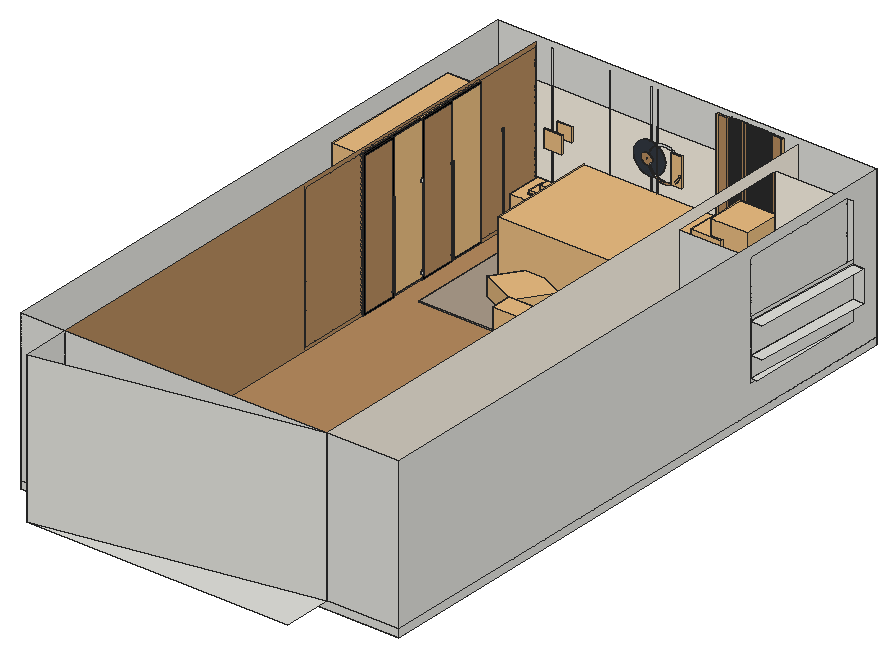
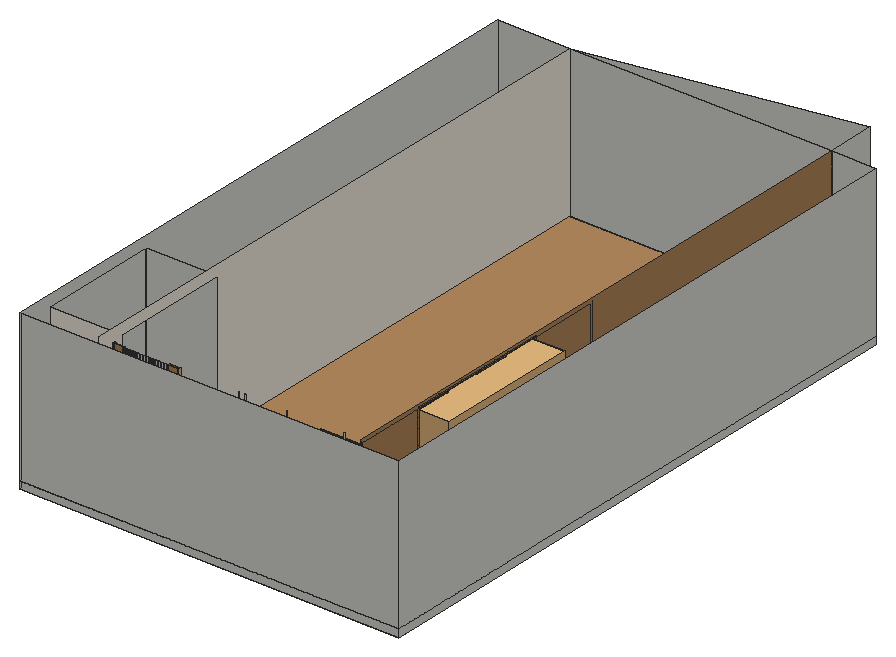
# SketchUp Ruby script. Lengths in inches.
U = 1.inch
M = Sketchup.active_model
def pt(a) = Geom::Point3d.new(a.map { |v| v * U })
def face(e, loops, mat)
  f = e.add_face(loops[0].map { |a| pt(a) })
  loops[1..].each { |l| e.add_face(l.map { |a| pt(a) }).erase! }
  f.material = f.back_material = mat if mat
  f
end
# faces: each face lists its corners as indices into pts; further lists are holes
def faces(e, pts, list, mat = nil) = list.each { |f| face(e, (f[0].is_a?(Array) ? f : [f]).map { |l| l.map { |i| pts[i] } }, mat) }
# xy, xz, yz: faces in a plane at the given z, y or x. An outline is a flat list of corners, or four numbers for a rectangle; further outlines are holes
def ring(l) = l.size == 4 ? [[l[0], l[1]], [l[2], l[1]], [l[2], l[3]], [l[0], l[3]]] : l.each_slice(2).to_a
def flat(e, list, mat, &to3) = list.each { |f| face(e, (f[0].is_a?(Array) ? f : [f]).map { |l| ring(l).map { |u, v| to3.(u, v) } }, mat) }
def xy(e, z, list, mat = nil) = flat(e, list, mat) { |x, y| [x, y, z] }
def xz(e, y, list, mat = nil) = flat(e, list, mat) { |x, z| [x, y, z] }
def yz(e, x, list, mat = nil) = flat(e, list, mat) { |y, z| [x, y, z] }
def lines(e, pts, list) = list.each { |a, b| e.add_line(pt(pts[a]), pt(pts[b])) }
# prism: a flat outline (further loops are holes) pulled along v
def prism(e, loops, v, mat = nil)
  f = face(e, loops, mat); d = Geom::Vector3d.new(v.map { |x| x * U })
  f.pushpull(f.normal.samedirection?(d) ? d.length : -d.length)
end
def box(e, o, s, mat = nil) = prism(e, [[o, [o[0] + s[0], o[1], o[2]], [o[0] + s[0], o[1] + s[1], o[2]], [o[0], o[1] + s[1], o[2]]]], [0, 0, s[2]], mat)
def at(x, y, z, deg = 0) = Geom::Transformation.translation(pt([x, y, z])) * Geom::Transformation.rotation(ORIGIN, Z_AXIS, deg.degrees)
def axes(o, x, y, z) = Geom::Transformation.new([*x, 0, *y, 0, *z, 0, *pt(o).to_a, 1])
def part(name) = M.definitions.add(name)
# library, detail: a bought-in or finely detailed component or shape, given as its bounding box
def library(name, o, s) = part(name).tap { |d| box(d.entities, o, s) }
def detail(e, o, s) = box(e.add_group.entities, o, s)
def put(e, d, t, mat = nil) = e.add_instance(d, t).tap { |i| i.material = mat if mat }
def group(e, t, mat = nil) = e.add_group.tap { |g| g.transformation = t; g.material = mat if mat }.entities
root = M.entities
M.materials.add("ChenZc-200606-DCZ97").color = [45, 44, 41]
M.materials.add("[0030_OldLace]").color = [253, 245, 230]
M.materials.add("[0110_LightSlateGray]").color = [51, 58, 66]
M.materials.add("[Color A01]").color = [254, 254, 199]
M.materials.add("[Color M09]").color = [0, 0, 0]
M.materials.add("[Metal_Aluminum_Anodized]1").color = [200, 209, 218]
M.materials.add("images-82sdfgh").color = [172, 157, 140]
M.materials.add("noyer1").color = [183, 140, 95]
c1 = library("组\#1",[0,0,0],[23.67,16.93,17.45])
c2 = library("Group22\#1",[-44.99,-22.85,-0.04],[43.91,45.38,19.57])
c3 = part("Untitled (22)")
g1 = group(c3.entities,at(0,0,0))
box(g1,[0,0,0],[170.08,120.47,0.79],"images-82sdfgh")
c4 = library("Group\#32",[-0.5,-0.5,0],[1,1.75,120])
c5 = library("Group\#33",[-0.5,-0.5,0],[1,1.9375,120])
c6 = library("Group\#27",[-9049.24,-32375.18,0],[19139.08,65939.34,16883.65])
c7 = part("27d7-b66a-ddc1-c0b1")
put(c7.entities,c6,at(0,0,0))
c8 = library("@05-床_01.第一季_组\#8",[0,0,0],[98.46,95.44,37.59])
c9 = library("Group80",[524.42,-273.19,102.05],[657.62,664.02,265.78])
c10 = library("Group73",[-242.83,-1394.05,-548.89],[487.85,171.35,750.9])
c11 = part("Дверь 1")
xy(c11.entities,0,[[0,-8.42,1.18,19.14]],"[Color M09]")
xy(c11.entities,0.79,[[0,-7.63,0.79,18.35],[0.79,-7.63,1.18,18.35]],"[Color M09]")
xy(c11.entities,95.67,[[0,-7.63,0.79,18.35]],"[Color M09]")
xy(c11.entities,95.67,[[0.79,-7.63,1.18,18.35]],"[Metal_Aluminum_Anodized]1")
xy(c11.entities,96.46,[[0,-8.42,1.18,19.14]],"[Color M09]")
xz(c11.entities,-8.42,[[0,0,1.18,96.46]],"[Color M09]")
xz(c11.entities,-7.63,[[0,0.79,0.79,95.67],[0.79,0.79,1.18,95.67]],"[Color M09]")
xz(c11.entities,18.35,[[0,0.79,0.79,95.67],[0.79,0.79,1.18,95.67]],"[Color M09]")
xz(c11.entities,19.14,[[0,0,1.18,96.46]],"[Metal_Aluminum_Anodized]1")
yz(c11.entities,0.79,[[-7.63,0.79,18.35,95.67]])
yz(c11.entities,1.18,[[[-8.42,0,19.14,96.46],[-7.63,0.79,18.35,95.67]]],"[Color M09]")
c12 = part("Group\#25")
put(c12.entities,c11,axes([0,38.03,0],[1,0,0],[0,1.05714,0],[0,0,1.11429]))
put(c12.entities,c11,axes([1.18,8.9,0],[1,0,0],[0,1.05714,0],[0,0,1.11429]))
c13 = library("dressing+1",[0,-1.62,0],[110.16,25.74,102.29])
c14 = part("POI-E1497-320-1917\#1")
xy(c14.entities,0,[[0,0,0.29,0.83],[7.21,0,7.5,0.83]])
xy(c14.entities,0.64,[[0.29,0.21,7.21,0.62]])
xy(c14.entities,0.875,[[0,0.21,7.5,0.62]])
xz(c14.entities,0.21,[[0,0.64,7.5,0.875]])
xz(c14.entities,0.62,[[0,0.64,7.5,0.875]])
yz(c14.entities,0,[[0,0,0.21,0.64,0.21,0.875,0.62,0.875,0.62,0.64,0.83,0]])
yz(c14.entities,0.29,[[0,0,0.83,0,0.62,0.64,0.21,0.64]])
yz(c14.entities,7.21,[[0,0,0.21,0.64,0.62,0.64,0.83,0]])
yz(c14.entities,7.5,[[0,0,0.83,0,0.62,0.64,0.62,0.875,0.21,0.875,0.21,0.64]])
p = [[0,0.21,0.64],[0,0,0],[0.29,0,0],[0.29,0.21,0.64],[7.21,0.21,0.64],[7.21,0,0],
  [7.5,0,0],[7.5,0.21,0.64],[0,0.83,0],[0,0.62,0.64],[0.29,0.62,0.64],[0.29,0.83,0],
  [7.5,0.83,0],[7.5,0.62,0.64],[7.21,0.62,0.64],[7.21,0.83,0]]
faces(c14.entities,p,[[0,1,2,3],[4,5,6,7],[8,9,10,11],[12,13,14,15]])
c15 = library("lamp",[0,0,0],[9.82,9.84,19.44])
c16 = library("17、植物花艺_花艺摆件_组\#4",[-0.13,-2.14,0],[21.63,21.46,31.4])
c17 = library("Pillow pair",[0,0,0],[18.27,24.9,18.7])
c18 = library("Group68\#1",[-167.83,-430.625,-1475.1875],[237.96,44,300])
c19 = library("Group69\#1",[-161.55,-462.88,-1311.24],[231.68,35.74,267.26])
c20 = library("Group67\#2",[-2553.52,-1371.9,-99.68],[199.61,250.46,199.36])
c21 = library("Omni Light",[-12,-12,-12],[24,24,24])
c22 = library("建立群組\#3",[-0.5,-0.5,0],[1.79,16.75,15.75])
c23 = library("Group\#29",[-0.5,-0.5,0],[8.5625,1,23.16])
c24 = library("建立群組\#4",[-0.5,-0.5,0],[1.79,16.75,15.75])
xy(root,-6,[[0,38.875,302.125,515.625]])
xy(root,0,[[35.9,0,244.6,38.875,244.6,0],[35.9,0,35.9,38.875,244.6,38.875],[0,38.875,35.9,38.875,35.9,508.85,48.54,508.85,48.54,508.97,48.84,508.97,48.84,508.85,94.41,508.85,94.41,508.97,94.71,508.97,94.71,508.85,127.66,508.85,127.66,508.97,127.96,508.97,127.96,508.85,132.6,508.85,132.6,508.97,132.9,508.97,132.9,508.85,180.6,508.85,180.6,509.54,189.03,509.54,189.03,509.85,190.82,509.85,190.82,510.22,191.46,510.22,191.46,509.85,193.25,509.85,193.25,510.22,193.9,510.22,193.9,509.85,195.69,509.85,195.69,510.22,196.34,510.22,196.34,509.85,198.13,509.85,198.13,510.22,198.78,510.22,198.78,509.85,200.57,509.85,200.57,510.22,201.21,510.22,201.21,509.85,203,509.85,203,510.22,203.53,510.22,203.53,509.85,205.32,509.85,205.32,510.22,205.84,510.22,205.84,509.85,207.63,509.85,207.63,510.22,208.15,510.22,208.15,509.85,209.94,509.85,209.94,510.22,210.46,510.22,210.46,509.85,212.25,509.85,212.25,510.22,212.78,510.22,212.78,509.85,214.57,509.85,214.57,510.22,215.09,510.22,215.09,509.85,216.88,509.85,216.88,510.22,217.4,510.22,217.4,509.85,219.19,509.85,219.19,510.22,219.71,510.22,219.71,509.85,221.5,509.85,221.5,510.22,222.03,510.22,222.03,509.85,223.82,509.85,223.82,510.22,224.53,510.22,224.53,509.54,232.6,509.54,232.6,508.85,244.6,508.85,244.6,38.875,302.125,38.875,302.125,515.625,0,515.625]])
xy(root,0,[[35.9,38.875,244.6,38.875,244.6,508.85,232.6,508.85,232.6,508.22,224.53,508.22,224.53,510.22,223.82,510.22,223.82,509.85,222.03,509.85,222.03,510.22,221.5,510.22,221.5,509.85,219.71,509.85,219.71,510.22,219.19,510.22,219.19,509.85,217.4,509.85,217.4,510.22,216.88,510.22,216.88,509.85,215.09,509.85,215.09,510.22,214.57,510.22,214.57,509.85,212.78,509.85,212.78,510.22,212.25,510.22,212.25,509.85,210.46,509.85,210.46,510.22,209.94,510.22,209.94,509.85,208.15,509.85,208.15,510.22,207.63,510.22,207.63,509.85,205.84,509.85,205.84,510.22,205.32,510.22,205.32,509.85,203.53,509.85,203.53,510.22,203,510.22,203,509.85,201.21,509.85,201.21,510.22,200.57,510.22,200.57,509.85,198.78,509.85,198.78,510.22,198.13,510.22,198.13,509.85,196.34,509.85,196.34,510.22,195.69,510.22,195.69,509.85,193.9,509.85,193.9,510.22,193.25,510.22,193.25,509.85,191.46,509.85,191.46,510.22,190.82,510.22,190.82,509.85,189.03,509.85,189.03,508.22,180.6,508.22,180.6,508.85,132.9,508.85,132.9,508.97,132.6,508.97,132.6,508.85,127.96,508.85,127.96,508.97,127.66,508.97,127.66,508.85,94.71,508.85,94.71,508.97,94.41,508.97,94.41,508.85,48.84,508.85,48.84,508.97,48.54,508.97,48.54,508.85,35.9,508.85],[180.6,508.22,189.03,509.54],[224.53,508.22,232.6,509.54]],"noyer1")
xy(root,3.11,[[2.53,335.23,35.9,450.62]],"noyer1")
xy(root,13.82,[[2.53,335.23,33.46,450.62]],"noyer1")
xy(root,14.91,[[2.53,335.23,33.46,450.62]],"noyer1")
xy(root,20.8125,[[244.6,390.22,244.91,486.22],[244.91,390.22,247.04,486.22]])
xy(root,21.9375,[[244.6,390.22,244.91,486.22],[244.91,390.22,247.04,486.22],[247.04,390.22,302.125,486.22]])
xy(root,25.1875,[[247.04,390.22,302.125,486.22],[302.125,390.22,302.125,486.22,306.875,486.22],[302.125,390.22,306.875,486.22,306.875,390.22]])
xy(root,37.91,[[2.53,335.23,33.46,450.62]],"noyer1")
xy(root,38.8,[[2.53,335.23,33.46,450.62]],"noyer1")
xy(root,41.64,[[311.68,389.75,302.125,390.22,306.875,486.22,316.43,485.75]])
xy(root,66.2,[[311.68,389.75,316.43,485.75,306.875,486.22,302.125,390.22]])
xz(root,38.875,[[0,-6,302.125,0],[0,0,35.9,120],[35.9,0,244.6,120],[244.6,0,302.125,120]])
xz(root,335.23,[[2.53,3.11,35.9,13.82],[2.53,13.82,33.46,14.91],[33.46,13.82,35.9,14.91],[2.53,14.91,35.9,37.91],[2.53,37.91,33.46,38.8],
  [33.46,37.91,35.9,38.8],[[2.53,38.8,35.9,85.91],[18.45,80.49,18.79,80.54,19.1,80.67,19.375,80.875,19.58,81.15,19.72,81.46,19.76,81.8,19.72,82.14,19.58,82.46,19.375,82.73,19.1,82.94,18.79,83.07,18.45,83.12,18.11,83.07,17.79,82.94,17.52,82.73,17.3125,82.46,17.18,82.14,17.14,81.8,17.18,81.46,17.3125,81.15,17.52,80.875,17.79,80.67,18.11,80.54]]])
xz(root,390.22,[[244.6,20.8125,244.91,21.9375],[244.91,20.8125,247.04,21.9375],[244.6,21.9375,244.6,25.1875,247.04,25.1875,246.71,25.04,246.41,24.86,246.12,24.66,245.84,24.43,245.59,24.17,245.37,23.9,245.17,23.61,245,23.3,244.85,22.97,244.74,22.63,244.65,22.29],[247.04,21.9375,302.125,25.1875],[244.6,25.1875,302.125,111.375]])
xz(root,450.62,[[2.53,3.11,35.9,13.82],[2.53,13.82,33.46,14.91],[33.46,13.82,35.9,14.91],[2.53,14.91,35.9,37.91],[2.53,37.91,33.46,38.8],
  [33.46,37.91,35.9,38.8],[[2.53,38.8,35.9,85.91],[18.45,80.49,18.11,80.54,17.79,80.67,17.52,80.875,17.3125,81.15,17.18,81.46,17.14,81.8,17.18,82.14,17.3125,82.46,17.52,82.73,17.79,82.94,18.11,83.07,18.45,83.12,18.79,83.07,19.1,82.94,19.375,82.73,19.58,82.46,19.72,82.14,19.76,81.8,19.72,81.46,19.58,81.15,19.375,80.875,19.1,80.67,18.79,80.54]]])
xz(root,486.22,[[244.6,20.8125,244.91,21.9375],[244.91,20.8125,247.04,21.9375],[247.04,21.9375,302.125,25.1875],[302.125,25.1875,306.875,111.375]])
xz(root,486.22,[[244.6,21.9375,244.65,22.29,244.74,22.63,244.85,22.97,245,23.3,245.17,23.61,245.37,23.9,245.59,24.17,245.84,24.43,246.12,24.66,246.41,24.86,246.71,25.04,247.04,25.1875,302.125,25.1875,302.125,111.375,244.6,111.375]],"[0030_OldLace]")
xz(root,506.41,[[[126.11,65.22,127.17,65.36,128.17,65.77,129.02,66.42,129.68,67.28,130.09,68.27,130.23,69.34,130.09,70.4,129.68,71.4,129.02,72.25,128.17,72.91,127.17,73.32,126.11,73.46,125.04,73.32,124.05,72.91,123.19,72.25,122.54,71.4,122.13,70.4,121.99,69.34,122.13,68.27,122.54,67.28,123.19,66.42,124.05,65.77,125.04,65.36],[125.18,68.71,126.7,70.22]]],"noyer1")
xz(root,507.33,[[126.11,65.22,125.04,65.36,124.05,65.77,123.19,66.42,122.54,67.28,122.13,68.27,121.99,69.34,122.13,70.4,122.54,71.4,123.19,72.25,124.05,72.91,125.04,73.32,126.11,73.46,126.26,73.4375,126.04,72.63,125.78,70.99,125.7,69.34,125.78,67.68,126.04,66.05,126.26,65.24],[126.26,65.24,126.04,66.05,125.78,67.68,125.7,69.34,125.78,70.99,126.04,72.63,126.26,73.4375,127.17,73.32,127.71,73.1,127.5,72.32,127.26,70.84,127.18,69.34,127.26,67.84,127.5,66.36,127.71,65.58,127.17,65.36],[127.71,65.58,127.5,66.36,127.26,67.84,127.18,69.34,127.26,70.84,127.5,72.32,127.71,73.1,128.17,72.91,129.02,72.25,129.68,71.4,130.09,70.4,130.23,69.34,130.09,68.27,129.68,67.28,129.02,66.42,128.17,65.77]])
xz(root,507.33,[[139.45,55.38,140.9,55.46,142.32,55.68,143.72,56.06,145.07,56.58,146.36,57.23,145.71,58.36,144.55,57.76,143.32,57.29,142.05,56.96,140.76,56.75,139.45,56.68,138.14,56.75,136.84,56.96,135.58,57.29,134.35,57.76,133.19,58.36,133.08,58.43,132.14,59.05,131.18,59.84,130.3,60.72,129.52,61.69,128.85,62.74,128.29,63.86,127.85,65.02,127.71,65.58,127.17,65.36,126.26,65.24,126.45,64.58,126.96,63.29,127.6,62.06,128.37,60.91,129.26,59.84,130.25,58.87,131.34,58.01,131.75,57.74,132.38,57.34,132.54,57.23,133.83,56.58,135.18,56.06,136.57,55.68,138,55.46]],"noyer1")
xz(root,508.04,[[139.45,55.38,138,55.46,136.57,55.68,135.18,56.06,133.83,56.58,132.54,57.23,132.38,57.34,131.75,57.74,131.81,57.76,132.98,58.36,133.08,58.43,133.19,58.36,134.35,57.76,135.58,57.29,136.84,56.96,138.14,56.75,139.45,56.68,140.76,56.75,142.05,56.96,143.32,57.29,144.55,57.76,145.71,58.36,146.8125,59.07,147.83,59.9,148.76,60.83,149.59,61.85,150.3,62.95,150.9,64.11,151.37,65.34,151.7,66.61,151.91,67.9,151.98,69.21,151.91,70.52,151.7,71.82,151.37,73.08,150.9,74.31,150.3,75.47,149.59,76.57,148.76,77.59,147.83,78.52,146.8125,79.35,145.71,80.06,144.55,80.66,143.32,81.125,142.05,81.47,140.76,81.67,139.45,81.74,138.14,81.67,136.84,81.47,135.58,81.125,134.35,80.66,133.19,80.06,133.08,79.99,132.98,80.06,131.81,80.66,131.75,80.68,132.38,81.08,132.54,81.1875,133.83,81.84,135.18,82.36,136.57,82.74,138,82.96,139.45,83.04,140.9,82.96,142.32,82.74,143.72,82.36,145.07,81.84,146.36,81.1875,147.58,80.4,148.7,79.49,149.73,78.46,150.64,77.34,151.43,76.125,152.08,74.83,152.6,73.48,152.98,72.09,153.2,70.66,153.28,69.21,153.2,67.76,152.98,66.34,152.6,64.9375,152.08,63.59,151.43,62.3,150.64,61.08,149.73,59.96,148.7,58.93,147.58,58.02,146.36,57.23,145.07,56.58,143.72,56.06,142.32,55.68,140.9,55.46]])
xz(root,508.04,[[126.72,56.68,128.03,56.75,129.32,56.96,130.59,57.29,131.75,57.74,131.32,58.02,130.2,58.93,129.17,59.96,128.26,61.08,127.47,62.3,126.82,63.59,126.3,64.9375,125.92,66.34,125.7,67.76,125.62,69.21,125.7,70.66,125.92,72.09,126.3,73.48,126.82,74.83,127.47,76.125,128.26,77.34,129.17,78.46,130.2,79.49,131.32,80.4,131.75,80.68,130.59,81.125,129.32,81.47,128.03,81.67,126.72,81.74,125.41,81.67,124.11,81.47,122.85,81.125,121.625,80.66,120.45,80.06,119.35,79.35,118.34,78.52,117.41,77.59,116.58,76.57,115.87,75.47,115.27,74.31,114.8,73.08,114.46,71.82,114.26,70.52,114.19,69.21,114.26,67.9,114.46,66.61,114.8,65.34,115.27,64.11,115.87,62.95,116.58,61.85,117.41,60.83,118.34,59.9,119.35,59.07,120.45,58.36,121.625,57.76,122.85,57.29,124.11,56.96,125.41,56.75],[133.08,58.43,134.08,59.07,135.1,59.9,136.03,60.83,136.85,61.85,137.57,62.95,138.16,64.11,138.63,65.34,138.97,66.61,139.18,67.9,139.25,69.21,139.18,70.52,138.97,71.82,138.63,73.08,138.16,74.31,137.57,75.47,136.85,76.57,136.03,77.59,135.1,78.52,134.08,79.35,133.08,79.99,132.09,79.35,131.07,78.52,130.14,77.59,129.3125,76.57,128.6,75.47,128,74.31,127.53,73.08,127.19,71.82,126.99,70.52,126.92,69.21,126.99,67.9,127.19,66.61,127.53,65.34,128,64.11,128.6,62.95,129.3125,61.85,130.14,60.83,131.07,59.9,132.09,59.07]],"[0110_LightSlateGray]")
xz(root,508.22,[[180.6,0,189.03,120],[224.53,0,232.6,120]],"noyer1")
xz(root,508.85,[[127.96,0,132.6,0,132.6,58.16,131.81,57.76,130.59,57.29,129.32,56.96,128.03,56.75,127.96,56.75],[126.72,56.68,127.66,56.73,127.66,81.69,126.72,81.74,125.41,81.67,124.11,81.47,122.85,81.125,121.625,80.66,120.45,80.06,119.35,79.35,118.34,78.52,117.41,77.59,116.58,76.57,115.87,75.47,115.27,74.31,114.8,73.08,114.46,71.82,114.26,70.52,114.19,69.21,114.26,67.9,114.46,66.61,114.8,65.34,115.27,64.11,115.87,62.95,116.58,61.85,117.41,60.83,118.34,59.9,119.35,59.07,120.45,58.36,121.625,57.76,122.85,57.29,124.11,56.96,125.41,56.75],[127.66,56.73,127.66,81.69,127.96,81.67,127.96,56.75],[127.96,56.75,128.03,56.75,129.32,56.96,130.59,57.29,131.81,57.76,132.6,58.16,132.6,80.26,131.81,80.66,130.59,81.125,129.32,81.47,128.03,81.67,127.96,81.67],[132.6,58.16,132.6,80.26,132.9,80.1,132.9,58.32],
  [132.9,58.32,132.9,80.1,132.98,80.06,134.08,79.35,135.1,78.52,136.03,77.59,136.85,76.57,137.57,75.47,138.16,74.31,138.63,73.08,138.97,71.82,139.18,70.52,139.25,69.21,139.18,67.9,138.97,66.61,138.63,65.34,138.16,64.11,137.57,62.95,136.85,61.85,136.03,60.83,135.1,59.9,134.08,59.07,132.98,58.36]])
xz(root,508.85,[[35.9,0,48.54,93.02],[48.84,0,94.41,93.02],[94.71,0,127.66,0,127.66,56.73,126.72,56.68,125.41,56.75,124.11,56.96,122.85,57.29,121.625,57.76,120.45,58.36,119.35,59.07,118.34,59.9,117.41,60.83,116.58,61.85,115.87,62.95,115.27,64.11,114.8,65.34,114.46,66.61,114.26,67.9,114.19,69.21,114.26,70.52,114.46,71.82,114.8,73.08,115.27,74.31,115.87,75.47,116.58,76.57,117.41,77.59,118.34,78.52,119.35,79.35,120.45,80.06,121.625,80.66,122.85,81.125,124.11,81.47,125.41,81.67,126.72,81.74,127.66,81.69,127.66,93.02,94.71,93.02],[132.9,0,180.6,0,180.6,93.02,132.9,93.02,132.9,80.1,132.98,80.06,134.08,79.35,135.1,78.52,136.03,77.59,136.85,76.57,137.57,75.47,138.16,74.31,138.63,73.08,138.97,71.82,139.18,70.52,139.25,69.21,139.18,67.9,138.97,66.61,138.63,65.34,138.16,64.11,137.57,62.95,136.85,61.85,136.03,60.83,135.1,59.9,134.08,59.07,132.98,58.36,132.9,58.32],[232.6,0,244.6,93.02]],"[0030_OldLace]")
xz(root,508.97,[[48.54,0,48.84,120],[94.41,0,94.71,120],[127.66,0,127.96,120],[132.6,0,132.9,120]])
xz(root,509.54,[[180.6,0,189.03,120],[224.53,0,232.6,120]],"noyer1")
xz(root,509.85,[[189.03,0,190.82,120],[191.46,0,193.25,120],[193.9,0,195.69,120],[196.34,0,198.13,120],[198.78,0,200.57,120],
  [201.21,0,203,120],[203.53,0,205.32,120],[205.84,0,207.63,120],[208.15,0,209.94,120],[210.46,0,212.25,120],
  [212.78,0,214.57,120],[215.09,0,216.88,120],[217.4,0,219.19,120],[219.71,0,221.5,120],[222.03,0,223.82,120]],"noyer1")
xz(root,510.22,[[190.82,0,191.46,120],[193.25,0,193.9,120],[195.69,0,196.34,120],[198.13,0,198.78,120],[200.57,0,201.21,120],
  [203,0,203.53,120],[205.32,0,205.84,120],[207.63,0,208.15,120],[209.94,0,210.46,120],[212.25,0,212.78,120],
  [214.57,0,215.09,120],[216.88,0,217.4,120],[219.19,0,219.71,120],[221.5,0,222.03,120],[223.82,0,224.53,120]],"noyer1")
xz(root,515.625,[[0,-6,302.125,0],[0,0,302.125,120]])
yz(root,0,[[38.875,-6,515.625,0],[38.875,0,515.625,120]])
yz(root,2.53,[[335.23,3.11,450.62,13.82],[335.23,13.82,450.62,14.91],[335.23,14.91,450.62,37.91],[335.23,37.91,450.62,38.8],[335.23,38.8,450.62,85.91]])
yz(root,33.46,[[335.23,13.82,450.62,14.91],[335.23,37.91,450.62,38.8]],"noyer1")
yz(root,35.9,[[0,0,38.875,120]])
yz(root,35.9,[[[38.875,0,508.85,0,508.85,93.02,508.97,93.02,508.97,93.32,508.85,93.32,508.85,120,38.875,120],[334.03,1.91,334.03,3.11,278.74,3.11,278.74,116.89,334.03,116.89,334.03,118.09,451.82,118.09,451.82,116.89,507.11,116.89,507.11,3.11,451.82,3.11,451.82,1.91]],[334.03,1.91,360.05,1.91,360.05,3.11,335.23,3.11,335.23,116.89,450.62,116.89,450.62,3.11,360.05,3.11,360.05,1.91,451.82,1.91,451.82,118.09,334.03,118.09],[278.74,3.11,334.03,116.89],[451.82,3.11,507.11,116.89]],"noyer1")
yz(root,48.54,[[508.85,0,508.97,93.02]])
yz(root,48.84,[[508.85,0,508.97,93.02]])
yz(root,94.41,[[508.85,0,508.97,93.02]])
yz(root,94.71,[[508.85,0,508.97,93.02]])
yz(root,127.66,[[508.85,0,508.97,93.02]])
yz(root,127.96,[[508.85,0,508.97,93.02]])
yz(root,132.6,[[508.85,0,508.97,93.02]])
yz(root,132.9,[[508.85,0,508.97,93.02]])
yz(root,180.6,[[508.85,0,508.85,93.02,508.97,93.02,508.97,93.32,508.85,93.32,508.85,120,509.54,120,509.54,0]])
yz(root,189.03,[[509.54,0,509.85,120]])
yz(root,189.03,[[508.22,0,509.54,120]],"noyer1")
yz(root,190.82,[[509.85,0,510.22,120]])
yz(root,191.46,[[509.85,0,510.22,120]])
yz(root,193.25,[[509.85,0,510.22,120]])
yz(root,193.9,[[509.85,0,510.22,120]])
yz(root,195.69,[[509.85,0,510.22,120]])
yz(root,196.34,[[509.85,0,510.22,120]])
yz(root,198.13,[[509.85,0,510.22,120]])
yz(root,198.78,[[509.85,0,510.22,120]])
yz(root,200.57,[[509.85,0,510.22,120]])
yz(root,201.21,[[509.85,0,510.22,120]])
yz(root,203,[[509.85,0,510.22,120]])
yz(root,203.53,[[509.85,0,510.22,120]])
yz(root,205.32,[[509.85,0,510.22,120]])
yz(root,205.84,[[509.85,0,510.22,120]])
yz(root,207.63,[[509.85,0,510.22,120]])
yz(root,208.15,[[509.85,0,510.22,120]])
yz(root,209.94,[[509.85,0,510.22,120]])
yz(root,210.46,[[509.85,0,510.22,120]])
yz(root,212.25,[[509.85,0,510.22,120]])
yz(root,212.78,[[509.85,0,510.22,120]])
yz(root,214.57,[[509.85,0,510.22,120]])
yz(root,215.09,[[509.85,0,510.22,120]])
yz(root,216.88,[[509.85,0,510.22,120]])
yz(root,217.4,[[509.85,0,510.22,120]])
yz(root,219.19,[[509.85,0,510.22,120]])
yz(root,219.71,[[509.85,0,510.22,120]])
yz(root,221.5,[[509.85,0,510.22,120]])
yz(root,222.03,[[509.85,0,510.22,120]])
yz(root,223.82,[[509.85,0,510.22,120]])
yz(root,224.53,[[509.54,0,510.22,120]])
yz(root,224.53,[[508.22,0,509.54,120]],"noyer1")
yz(root,232.6,[[508.85,0,509.54,0,509.54,120,508.85,120,508.85,93.32,509.16,93.32,509.16,93.02,508.85,93.02]])
yz(root,244.6,[[[38.875,0,38.875,120,508.85,120,508.85,93.32,509.16,93.32,509.16,93.02,508.85,93.02,508.85,0],[390.22,20.8125,486.22,111.375]]],"[0030_OldLace]")
yz(root,244.91,[[390.22,20.8125,486.22,21.9375]])
yz(root,247.04,[[390.22,20.8125,486.22,21.9375],[390.22,21.9375,486.22,25.1875]])
yz(root,302.125,[[38.875,-6,515.625,0],[[38.875,0,515.625,120],[390.22,21.9375,486.22,111.375]],[390.22,21.9375,486.22,25.1875],[390.22,25.1875,486.22,111.375]])
p = [[35.9,0,0],[244.6,38.875,0],[244.6,38.875,120],[35.9,0,120],[244.65,486.22,22.29],[244.6,486.22,21.9375],
  [244.6,390.22,21.9375],[244.65,390.22,22.29],[244.74,486.22,22.63],[244.74,390.22,22.63],[244.85,486.22,22.97],[244.85,390.22,22.97],
  [245,486.22,23.3],[245,390.22,23.3],[245.17,486.22,23.61],[245.17,390.22,23.61],[245.37,486.22,23.9],[245.37,390.22,23.9],
  [245.59,486.22,24.17],[245.59,390.22,24.17],[245.84,486.22,24.43],[245.84,390.22,24.43],[246.12,486.22,24.66],[246.12,390.22,24.66],
  [246.41,486.22,24.86],[246.41,390.22,24.86],[246.71,486.22,25.04],[246.71,390.22,25.04],[247.04,486.22,25.1875],[247.04,390.22,25.1875],
  [302.125,390.22,25.1875],[306.875,486.22,25.1875],[306.875,486.22,41.64],[302.125,390.22,41.64],[306.875,486.22,66.2],[302.125,390.22,66.2],
  [316.43,485.75,66.2],[316.43,485.75,41.64],[138,508.04,55.46],[139.45,508.04,55.38],[139.45,507.33,55.38],[138,507.33,55.46],
  [140.9,508.04,55.46],[140.9,507.33,55.46],[136.57,508.04,55.68],[136.57,507.33,55.68],[142.32,508.04,55.68],[142.32,507.33,55.68],
  [135.18,508.04,56.06],[135.18,507.33,56.06],[143.72,508.04,56.06],[143.72,507.33,56.06],[133.83,508.04,56.58],[133.83,507.33,56.58],
  [145.07,508.04,56.58],[145.07,507.33,56.58],[132.54,508.04,57.23],[132.54,507.33,57.23],[146.36,508.04,57.23],[146.36,507.33,57.23],
  [139.45,508.04,56.68],[138.14,508.04,56.75],[138.14,507.33,56.75],[139.45,507.33,56.68],[140.76,508.04,56.75],[140.76,507.33,56.75],
  [125.41,508.85,56.75],[126.72,508.85,56.68],[126.72,508.04,56.68],[125.41,508.04,56.75],[127.96,508.85,56.75],[128.03,508.85,56.75],
  [128.03,508.04,56.75],[127.66,508.85,56.73],[136.84,508.04,56.96],[136.84,507.33,56.96],[142.05,508.04,56.96],[142.05,507.33,56.96],
  [124.11,508.85,56.96],[124.11,508.04,56.96],[129.32,508.85,56.96],[129.32,508.04,56.96],[135.58,508.04,57.29],[135.58,507.33,57.29],
  [143.32,508.04,57.29],[143.32,507.33,57.29],[122.85,508.85,57.29],[122.85,508.04,57.29],[130.59,508.85,57.29],[130.59,508.04,57.29],
  [132.38,508.04,57.34],[132.38,507.33,57.34],[147.58,508.04,58.02],[147.58,507.33,58.02],[131.75,508.04,57.74],[131.75,507.33,57.74],
  [134.35,508.04,57.76],[134.35,507.33,57.76],[144.55,508.04,57.76],[144.55,507.33,57.76],[121.625,508.85,57.76],[121.625,508.04,57.76],
  [131.81,508.85,57.76],[131.81,508.04,57.76],[131.34,507.33,58.01],[131.32,508.04,58.02],[133.19,508.04,58.36],[133.19,507.33,58.36],
  [145.71,508.04,58.36],[145.71,507.33,58.36],[120.45,508.85,58.36],[120.45,508.04,58.36],[132.98,508.85,58.36],[132.98,508.04,58.36],
  [132.6,508.85,58.16],[132.9,508.85,58.32],[130.25,507.33,58.87],[130.2,508.04,58.93],[148.7,508.04,58.93],[148.7,507.33,58.93],
  [132.14,507.33,59.05],[133.08,507.33,58.43],[132.09,508.04,59.07],[133.08,508.04,58.43],[146.8125,508.04,59.07],[146.8125,507.33,59.07],
  [119.35,508.85,59.07],[119.35,508.04,59.07],[134.08,508.04,59.07],[134.08,508.85,59.07],[129.17,508.04,59.96],[129.26,507.33,59.84],
  [149.73,508.04,59.96],[149.73,507.33,59.96],[131.07,508.04,59.9],[131.18,507.33,59.84],[147.83,508.04,59.9],[147.83,507.33,59.9],
  [118.34,508.85,59.9],[118.34,508.04,59.9],[135.1,508.85,59.9],[135.1,508.04,59.9],[128.37,507.33,60.91],[128.26,508.04,61.08],
  [130.3,507.33,60.72],[130.14,508.04,60.83],[148.76,508.04,60.83],[148.76,507.33,60.83],[117.41,508.85,60.83],[117.41,508.04,60.83],
  [136.03,508.85,60.83],[136.03,508.04,60.83],[150.64,508.04,61.08],[150.64,507.33,61.08],[129.52,507.33,61.69],[129.3125,508.04,61.85],
  [149.59,508.04,61.85],[149.59,507.33,61.85],[116.58,508.85,61.85],[116.58,508.04,61.85],[136.85,508.85,61.85],[136.85,508.04,61.85],
  [127.6,507.33,62.06],[127.47,508.04,62.3],[151.43,508.04,62.3],[151.43,507.33,62.3],[128.85,507.33,62.74],[128.6,508.04,62.95],
  [150.3,508.04,62.95],[150.3,507.33,62.95],[115.87,508.85,62.95],[115.87,508.04,62.95],[137.57,508.85,62.95],[137.57,508.04,62.95],
  [126.96,507.33,63.29],[126.82,508.04,63.59],[152.08,508.04,63.59],[152.08,507.33,63.59],[128.29,507.33,63.86],[128,508.04,64.11],
  [150.9,508.04,64.11],[150.9,507.33,64.11],[115.27,508.85,64.11],[115.27,508.04,64.11],[138.16,508.85,64.11],[138.16,508.04,64.11],
  [126.45,507.33,64.58],[126.3,508.04,64.9375],[152.6,508.04,64.9375],[152.6,507.33,64.9375],[127.85,507.33,65.02],[127.53,508.04,65.34],
  [151.37,508.04,65.34],[151.37,507.33,65.34],[114.8,508.85,65.34],[114.8,508.04,65.34],[138.63,508.85,65.34],[138.63,508.04,65.34],
  [126.26,507.33,65.24],[125.92,508.04,66.34],[152.98,508.04,66.34],[152.98,507.33,66.34],[127.71,507.33,65.58],[125.04,507.33,65.36],
  [126.11,507.33,65.22],[126.11,506.41,65.22],[125.04,506.41,65.36],[127.17,507.33,65.36],[127.17,506.41,65.36],[126.04,507.33,66.05],
  [127.19,508.04,66.61],[127.5,507.33,66.36],[151.7,508.04,66.61],[151.7,507.33,66.61],[114.46,508.85,66.61],[114.46,508.04,66.61],
  [138.97,508.85,66.61],[138.97,508.04,66.61],[124.05,507.33,65.77],[124.05,506.41,65.77],[128.17,507.33,65.77],[128.17,506.41,65.77],
  [123.19,507.33,66.42],[123.19,506.41,66.42],[129.02,507.33,66.42],[129.02,506.41,66.42],[125.78,507.33,67.68],[125.7,508.04,67.76],
  [306.875,486.22,69.25],[302.125,390.22,69.25],[153.2,508.04,67.76],[153.2,507.33,67.76],[122.54,507.33,67.28],[122.54,506.41,67.28],
  [129.68,507.33,67.28],[129.68,506.41,67.28],[126.99,508.04,67.9],[127.26,507.33,67.84],[151.91,508.04,67.9],[151.91,507.33,67.9],
  [114.26,508.85,67.9],[114.26,508.04,67.9],[139.18,508.85,67.9],[139.18,508.04,67.9],[35.9,277.53,118.09],[35.9,277.53,1.91],
  [35.9,508.32,118.09],[35.9,508.32,1.91]]
faces(root,p,[[0,1,2,3],[30,31,32,33],[34,35,33,32],[32,34,36,37],[38,39,40,41],[39,42,43,40],[44,38,41,45],[42,46,47,43],
  [48,44,45,49],[46,50,51,47],[52,48,49,53],[50,54,55,51],[56,52,53,57],[54,58,59,55],[60,61,62,63],[64,60,63,65],
  [66,67,68,69],[70,71,72,68,67,73],[61,74,75,62],[76,64,65,77],[78,66,69,79],[71,80,81,72],[74,82,83,75],[84,76,77,85],
  [86,78,79,87],[80,88,89,81],[90,56,57,91],[58,92,93,59],[94,90,91,95],[82,96,97,83],[98,84,85,99],[100,86,87,101],
  [102,103,94,89,88],[95,104,94],[105,94,104],[96,106,107,97],[108,98,99,109],[110,100,101,111],[112,113,103,102,114,115],[104,116,105],
  [117,105,116],[92,118,119,93],[120,121,122],[123,122,121],[121,107,106,123],[124,108,109,125],[126,110,111,127],[128,123,113,112,129],
  [130,117,131],[116,131,117],[118,132,133,119],[122,134,120],[135,120,134],[136,124,125,137],[138,126,127,139],[129,140,141,128],
  [142,143,131],[130,131,143],[144,135,145],[134,145,135],[146,136,137,147],[148,138,139,149],[140,150,151,141],[132,152,153,133],
  [144,145,154],[155,154,145],[156,146,147,157],[158,148,149,159],[150,160,161,151],[162,163,142],[143,142,163],[152,164,165,153],
  [154,155,166],[167,166,155],[168,156,157,169],[170,158,159,171],[160,172,173,161],[174,175,162],[163,162,175],[164,176,177,165],
  [166,167,178],[179,178,167],[180,168,169,181],[182,170,171,183],[172,184,185,173],[186,187,174],[175,174,187],[176,188,189,177],
  [178,179,190],[191,190,179],[192,180,181,193],[194,182,183,195],[184,196,197,185],[186,198,199],[187,186,199],[188,200,201,189],
  [190,191,202],[203,204,205,206],[198,207,208,205,204],[209,199,198],[202,191,210,211],[212,192,193,213],[214,194,195,215],[196,216,217,197],
  [218,203,206,219],[202,220,221,208,207],[222,218,219,223],[220,224,225,221],[226,227,199,209],[228,229,35,34],[200,230,231,201],[232,222,223,233],
  [224,234,235,225],[211,210,236,237],[238,212,213,239],[240,214,215,241],[216,242,243,217]])
faces(root,p,[[4,5,6,7],[8,4,7,9],[10,8,9,11],[12,10,11,13],[14,12,13,15],[16,14,15,17],[18,16,17,19],[20,18,19,21],
  [22,20,21,23],[24,22,23,25],[26,24,25,27],[28,26,27,29]],"[0030_OldLace]")
lines(root,p,[[244,245],[246,247]])
put(root,c1,axes([41.55,475.98,0],[1.61138,0,0],[0,1.61138,0],[0,0,1.61138]))
put(root,c1,axes([190.6875,478,0],[1.50742,0,0],[0,1.50742,0],[0,0,1.50742]))
put(root,c2,axes([270.27,425.72,0.0625],[1,0,0],[0,1.56,0],[0,0,1.50134]),"[0030_OldLace]")
put(root,c3,axes([51.82,371.64,0],[1,0,0],[0,0.83,0],[0,0,1]))
put(root,c4,at(180.6,508.22,0))
put(root,c5,at(232.6,508.22,0))
g2 = group(root,at(174.98,409.87,0.73))
xy(g2,0,[[-1.87,-1.95,1.87,1.95]],"ChenZc-200606-DCZ97")
xy(g2,1.84,[[-2.125,-2.22,2.125,2.22]],"ChenZc-200606-DCZ97")
p = [[2.125,-2.22,1.84],[1.87,-1.95,0],[-1.87,-1.95,0],[-2.125,-2.22,1.84],[-1.87,1.95,0],[-2.125,2.22,1.84],
  [2.125,2.22,1.84],[1.87,1.95,0]]
faces(g2,p,[[0,1,2,3],[3,2,4,5],[6,7,1,0],[5,4,7,6]],"ChenZc-200606-DCZ97")
put(root,c7,axes([143.71,380.01,0.79],[0,-0.00083,0],[0.001,0,0],[0,0,0.001]))
put(root,c8,axes([74.22,422.74,0.99],[1.19825,0,0],[0,0.95476,0],[0,0,1.19825]))
put(root,c9,axes([148.3,390.53,-4.19],[-0.04725,0.02264,0],[-0.02728,-0.03922,0],[0,0,0.05456]))
put(root,c10,axes([186.62,414.37,75.19],[-0.02233,0.03974,0],[0,0,0.05283],[0.04788,0.01853,0]))
put(root,c12,axes([35.9,392.55,1.91],[1,0,0],[0,1.01721,0],[0,0,1.07]),"noyer1")
put(root,c12,axes([35.9,334.29,1.91],[1,0,0],[0,1,0],[0,0,1.07]),"noyer1")
put(root,c13,axes([35.9,335.23,3.11],[0,1.0457,0],[-1,0,0],[0,0,1.09774]))
put(root,c14,axes([35.9,474.125,74.23],[0,0,-9.12],[0,1.13818,0],[2.0064,0,0]))
put(root,c14,axes([37.87,421.34,74.64],[0,0,-9.12],[0,1.13818,0],[2.0064,0,0]))
put(root,c14,axes([37.87,391.72,74.64],[0,0,-9.12],[0,1.13818,0],[2.0064,0,0]))
put(root,c14,axes([37.87,362.59,74.64],[0,0,-9.12],[0,1.13818,0],[2.0064,0,0]))
put(root,c15,axes([193.07,476.68,24.01],[1.4985,0,0],[0,1.4985,0],[0,0,1.1988]))
put(root,c16,axes([203.13,477.2,24.66],[1.37175,0,0],[0,1.37175,0],[0,0,1.37175]))
put(root,c17,at(264.57,462.98,24.86,55),"[0030_OldLace]")
put(root,c18,axes([-27.32,486.63,46.81],[0,-0.05838,0],[0,0,0.04741],[-0.06607,0,0]))
put(root,c19,axes([-27.26,487.57,48.52],[0,-0.05334,0],[0,0,0.04323],[-0.07433,0,0]))
put(root,c20,axes([-34.6875,491.33,52.11],[-0.03847,0,0],[0,0,0.01605],[0,-0.03864,0]))
put(root,c21,at(200.59,483.92,43.9))
put(root,c22,axes([52.75,497.05,55.71],[0,-0.85,0],[0.85,0,0],[0,0,0.85]),"[Color A01]")
put(root,c23,at(145.71,507.33,57.23))
put(root,c24,axes([60.54,500.03,64.93],[0,-0.70766,0],[0.70766,0,0],[0,0,0.70766]),"[Color A01]")
